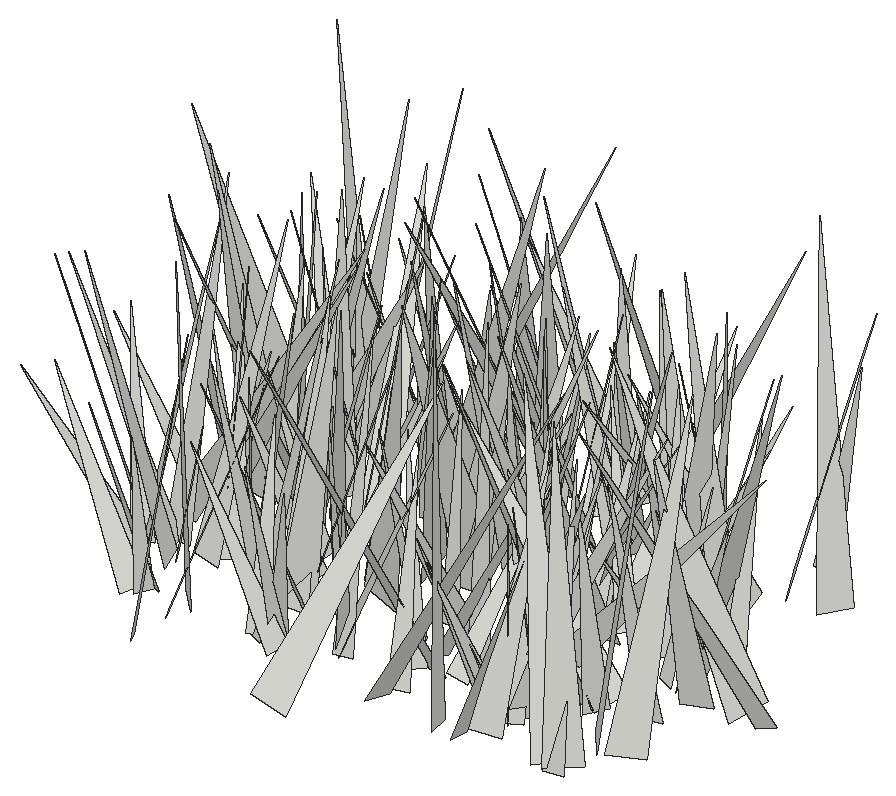
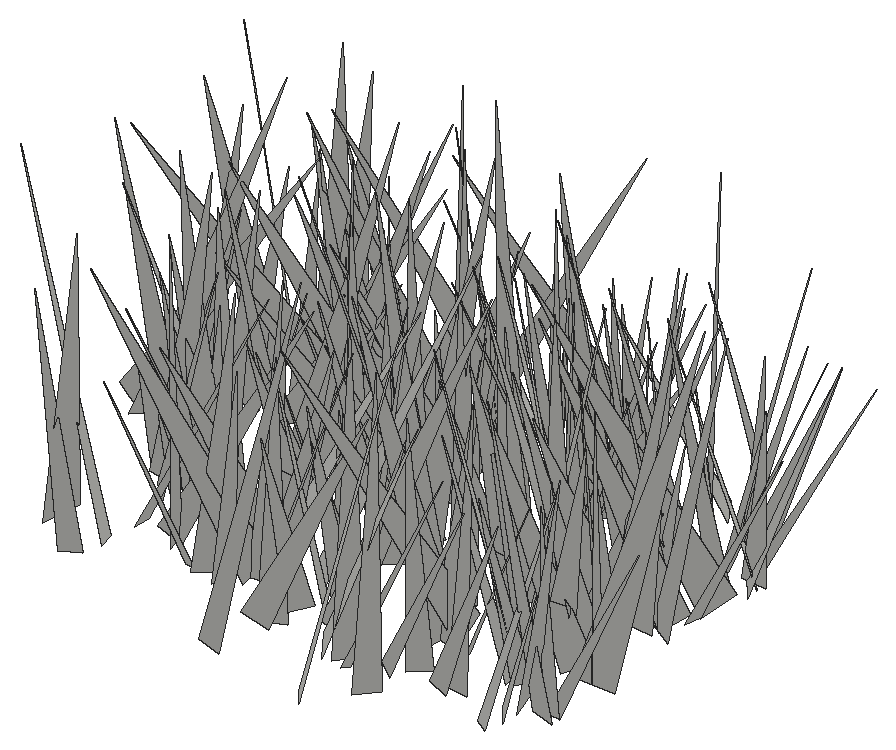
# SketchUp Ruby script. Lengths in inches.
U = 1.inch
M = Sketchup.active_model
def pt(a) = Geom::Point3d.new(a.map { |v| v * U })
def face(e, loops, mat)
  f = e.add_face(loops[0].map { |a| pt(a) })
  loops[1..].each { |l| e.add_face(l.map { |a| pt(a) }).erase! }
  f.material = f.back_material = mat if mat
  f
end
# faces: each face lists its corners as indices into pts; further lists are holes
def faces(e, pts, list, mat = nil) = list.each { |f| face(e, (f[0].is_a?(Array) ? f : [f]).map { |l| l.map { |i| pts[i] } }, mat) }
# xy, xz, yz: faces in a plane at the given z, y or x. An outline is a flat list of corners, or four numbers for a rectangle; further outlines are holes
def ring(l) = l.size == 4 ? [[l[0], l[1]], [l[2], l[1]], [l[2], l[3]], [l[0], l[3]]] : l.each_slice(2).to_a
def flat(e, list, mat, &to3) = list.each { |f| face(e, (f[0].is_a?(Array) ? f : [f]).map { |l| ring(l).map { |u, v| to3.(u, v) } }, mat) }
def xy(e, z, list, mat = nil) = flat(e, list, mat) { |x, y| [x, y, z] }
def xz(e, y, list, mat = nil) = flat(e, list, mat) { |x, z| [x, y, z] }
def yz(e, x, list, mat = nil) = flat(e, list, mat) { |y, z| [x, y, z] }
def lines(e, pts, list) = list.each { |a, b| e.add_line(pt(pts[a]), pt(pts[b])) }
# prism: a flat outline (further loops are holes) pulled along v
def prism(e, loops, v, mat = nil)
  f = face(e, loops, mat); d = Geom::Vector3d.new(v.map { |x| x * U })
  f.pushpull(f.normal.samedirection?(d) ? d.length : -d.length)
end
def box(e, o, s, mat = nil) = prism(e, [[o, [o[0] + s[0], o[1], o[2]], [o[0] + s[0], o[1] + s[1], o[2]], [o[0], o[1] + s[1], o[2]]]], [0, 0, s[2]], mat)
def at(x, y, z, deg = 0) = Geom::Transformation.translation(pt([x, y, z])) * Geom::Transformation.rotation(ORIGIN, Z_AXIS, deg.degrees)
def axes(o, x, y, z) = Geom::Transformation.new([*x, 0, *y, 0, *z, 0, *pt(o).to_a, 1])
def part(name) = M.definitions.add(name)
# library, detail: a bought-in or finely detailed component or shape, given as its bounding box
def library(name, o, s) = part(name).tap { |d| box(d.entities, o, s) }
def detail(e, o, s) = box(e.add_group.entities, o, s)
def put(e, d, t, mat = nil) = e.add_instance(d, t).tap { |i| i.material = mat if mat }
def group(e, t, mat = nil) = e.add_group.tap { |g| g.transformation = t; g.material = mat if mat }.entities
root = M.entities
c1 = part("fur_instance\#9")
p = [[0.8125,0,1.79],[0.67,-0.02,1.48],[0,-0.11,0],[0,0.11,0]]
faces(c1.entities,p,[[0,1,2,3]])
put(root,c1,axes([468.71,19.62,-21.86],[-0.73588,7.38124,0.25307],[6.98236,0.77818,-2.39362],[2.40696,-0.00075,7.02103]))
put(root,c1,axes([461.41,20.5,-21.86],[4.53649,3.63122,1.57008],[3.09166,-4.74451,2.04009],[-2.46831,0.73111,5.44092]))
put(root,c1,axes([466.3,23.18,-21.86],[-4.45422,0.97791,0.2811],[1.01486,4.3608,0.91044],[0.07343,-0.95002,4.4685]))
put(root,c1,axes([465.92,23.8125,-21.86],[-3.9744,-0.24759,1.6573],[0.13335,4.20562,0.94807],[1.67038,-0.92483,3.8676]))
put(root,c1,axes([459.53,23.55,-21.86],[2.92591,-1.89098,1.19539],[-1.88086,-3.14489,-0.37117],[-1.21125,0.31559,3.46396]))
put(root,c1,axes([465.51,24.1875,-21.86],[0.57309,-4.07864,0.58369],[-4.03575,-0.43699,0.90892],[0.82985,0.69149,4.01716]))
put(root,c1,axes([459.61,24.03,-21.86],[-2.05359,-3.75931,0.63579],[-3.81243,2.01617,-0.39286],[-0.04503,0.74602,4.26559]))
put(root,c1,axes([480.43,22.82,-21.86],[-4.52139,5.22079,2.42729],[5.56937,4.74843,0.161],[1.45961,-1.94607,6.90462]))
put(root,c1,axes([459.09,23.44,-21.86],[-3.88022,2.75048,0.41463],[2.75578,3.70465,1.21426],[-0.37781,-1.22622,4.59857]))
put(root,c1,axes([461.28,24.04,-21.86],[-4.9247,-5.05159,2.9073],[-5.39927,5.38751,0.21521],[2.19519,1.91829,7.05159]))
put(root,c1,axes([472.15,25.59,-21.86],[-3.80092,-6.72254,0.0507],[-6.48684,3.65215,-2.05545],[-1.76524,1.05421,7.4441]))
put(root,c1,axes([474.72,22.4,-21.86],[-7.45834,-2.27512,2.73301],[-2.96816,7.48025,-1.87304],[1.95846,2.67246,7.56933]))
put(root,c1,axes([476.37,24.59,-21.86],[-3.42009,-2.62307,1.97794],[-2.56254,3.91671,0.76324],[2.05575,0.51835,4.24205]))
put(root,c1,axes([479.86,22.92,-21.86],[-6.04844,4.67756,1.28768],[4.75602,6.12308,0.0974],[0.95811,-0.86582,7.6455]))
put(root,c1,axes([468,25.06,-21.86],[3.91592,-0.46866,0.80636],[-0.26131,-3.89224,-0.99321],[-0.89531,-0.91384,3.81675]))
put(root,c1,axes([476.48,23.02,-21.86],[-2.07384,5.25709,1.74566],[5.26815,2.4479,-1.11335],[1.712,-1.16445,5.54061]))
put(root,c1,axes([480.41,22.25,-21.86],[1.19098,5.93826,0.851],[5.76454,-1.37303,1.51343],[-1.66049,-0.50738,5.86438]))
put(root,c1,axes([474.43,25.75,-21.86],[-3.37943,-0.96857,0.84627],[-0.6019,3.29348,1.36586],[1.13667,-1.13567,3.23931]))
put(root,c1,axes([465.04,23.63,-21.86],[-1.62337,4.08317,1.17277],[4.21606,1.70273,-0.09236],[0.52201,-1.05424,4.39307]))
put(root,c1,axes([474.19,25.72,-21.86],[0.37183,-3.94608,0.38846],[-3.8933,-0.43727,-0.71534],[-0.75144,0.31297,3.89847]))
put(root,c1,axes([457.46,26.01,-21.86],[-4.70731,-0.314,0.0439],[-0.28456,4.4722,1.47573],[0.13983,-1.46975,4.48103]))
put(root,c1,axes([471.54,22.68,-21.86],[7.73901,0.54751,0.09462],[0.50511,-7.48314,1.98706],[-0.23147,1.9758,7.49957]))
put(root,c1,axes([475.8125,22.29,-21.86],[6.82922,2.21825,1.16198],[1.82522,-6.72015,2.10172],[-1.71447,1.68168,6.86597]))
put(root,c1,axes([471.79,23.63,-21.86],[-0.43977,4.5707,0.64422],[4.59918,0.3789,0.45132],[-0.39225,-0.6818,4.56957]))
put(root,c1,axes([461.29,22.77,-21.86],[4.51704,3.2359,0.24642],[3.07452,-4.40221,1.45028],[-1.0388,1.04161,5.3639]))
put(root,c1,axes([458.77,26.14,-21.86],[-6.28754,-2.52373,1.27093],[-2.51372,6.41179,0.29625],[1.29062,0.19325,6.76865]))
put(root,c1,axes([468,24.81,-21.86],[4.98455,3.49636,0.32674],[3.50629,-4.92427,-0.79656],[0.19289,-0.83908,6.03621]))
put(root,c1,axes([480.18,25.12,-21.86],[5.88152,4.86813,2.28116],[5.13014,-6.09312,-0.22398],[-1.60749,-1.63397,7.63157]))
put(root,c1,axes([463.08,26.35,-21.86],[-4.89796,-0.50596,1.28828],[-0.38248,5.0478,0.52832],[1.33018,-0.4116,4.8956]))
put(root,c1,axes([458.69,26.64,-21.86],[3.46775,1.51161,0.84573],[1.722,-3.21287,-1.3182],[-0.18693,-1.55498,3.54578]))
put(root,c1,axes([464.76,26.21,-21.86],[2.84119,-6.18581,2.36185],[-6.62137,-2.65127,1.02137],[0.00779,2.57322,6.73004]))
put(root,c1,axes([467.27,25.84,-21.86],[1.82668,3.73793,1.95155],[3.99067,-2.21946,0.51574],[-1.36206,-1.48974,4.1283]))
put(root,c1,axes([476.17,26.43,-21.86],[-3.08736,-2.6391,1.38175],[-2.74426,3.29386,0.15946],[1.15895,0.7691,4.05847]))
put(root,c1,axes([464.96,23.41,-21.86],[4.10406,6.33899,0.98584],[6.11766,-4.2195,1.66374],[-1.93105,0.10466,7.36601]))
put(root,c1,axes([465.36,26.02,-21.86],[-3.16767,-3.69393,0.44061],[-3.42422,2.66901,-2.24153],[-1.45395,1.76199,4.31912]))
put(root,c1,axes([478.11,27.0625,-21.86],[-4.08084,-6.31933,0.93728],[-6.28934,3.77891,-1.90517],[-1.12095,1.80323,7.27719]))
put(root,c1,axes([470.4,26.77,-21.86],[-4.55771,-1.35516,1.4154],[-1.26006,4.77117,0.51063],[1.50069,-0.10962,4.72742]))
put(root,c1,axes([471.85,28.2,-21.86],[1.26749,-5.25605,0.55346],[-5.00773,-1.37633,-1.60227],[-1.68968,0.13629,5.16385]))
put(root,c1,axes([476.68,24.78,-21.86],[4.97283,-0.90694,1.68915],[-1.45035,-4.85051,1.66547],[-1.25389,2.01364,4.77261]))
put(root,c1,axes([478.7,26.98,-21.86],[3.6689,-2.8215,1.45683],[-2.81207,-3.92099,-0.512],[-1.47496,0.45716,4.59995]))
put(root,c1,axes([470.6875,24.8125,-21.86],[5.2038,5.70361,2.35891],[5.67233,-5.63566,1.11317],[-2.43315,-0.93989,7.64013]))
put(root,c1,axes([474.21,28.54,-21.86],[1.01842,-6.5564,0.3467],[-5.92672,-0.76709,2.90332],[2.82498,0.75429,5.9661]))
put(root,c1,axes([466.95,28.66,-21.86],[-0.13317,-8.12567,1.45261],[-7.87911,0.55826,2.40046],[2.46092,1.34765,7.76415]))
put(root,c1,axes([468.55,24.32,-21.86],[1.43264,6.02249,0.66756],[5.77311,-1.565,1.72927],[-1.84042,-0.22107,5.94411]))
put(root,c1,axes([471.28,25.3125,-21.86],[-4.35702,1.54483,0.37411],[1.45493,4.3157,-0.87633],[0.64002,0.7059,4.53896]))
put(root,c1,axes([476.74,24.23,-21.86],[-5.37291,2.30629,0.61766],[1.96946,5.14098,-2.06404],[1.34972,1.6793,5.47055]))
put(root,c1,axes([457.12,26.87,-21.86],[-4.61833,-3.74237,0.73758],[-3.79853,4.40694,-1.4242],[-0.34716,1.56584,5.77113]))
put(root,c1,axes([476.65,26.6875,-21.86],[2.40837,2.51325,1.53163],[2.71206,-2.66382,0.10655],[-1.14326,-1.0248,3.47927]))
put(root,c1,axes([481.76,24.96,-21.86],[-4.86903,5.31705,1.90275],[5.12727,5.21523,-1.45307],[2.36698,-0.35954,7.06166]))
put(root,c1,axes([464.75,25.98,-21.86],[-0.45657,6.34549,1.8425],[6.59681,0.54314,-0.23589],[0.37708,-1.81886,6.35752]))
put(root,c1,axes([458.1875,27.12,-21.86],[-6.00367,-1.40851,0.07652],[-1.40991,5.98159,-0.51624],[-0.04369,0.52005,6.14503]))
put(root,c1,axes([464.02,28.47,-21.86],[-4.35378,0.44066,1.23045],[0.84047,4.2213,1.46212],[1.0009,-1.62788,4.12453]))
put(root,c1,axes([461.8,27.29,-21.86],[3.22406,2.21993,1.84513],[2.48282,-3.54361,-0.0749],[-1.47248,-1.11442,3.91371]))
put(root,c1,axes([480.71,27.74,-21.86],[-0.10037,-5.00985,1.67679],[-5.24561,-0.10471,-0.62683],[-0.62754,1.67652,4.9715]))
put(root,c1,axes([478.71,27.92,-21.86],[-6.39943,2.86094,0.01202],[2.71801,6.07041,2.2137],[-0.89308,-2.0256,6.65111]))
put(root,c1,axes([475.84,25.44,-21.86],[5.89458,-2.32049,1.52507],[-2.76984,-5.16651,2.8446],[-0.1962,3.22166,5.6603]))
put(root,c1,axes([457.125,26.49,-21.86],[-0.91318,4.58049,0.90258],[4.61205,0.74242,0.89849],[-0.72428,-1.04754,4.5834]))
put(root,c1,axes([472.99,25.71,-21.86],[-0.63847,4.33122,0.11328],[4.14955,0.64421,-1.24344],[1.2464,0.07394,4.19773]))
put(root,c1,axes([475.76,26.43,-21.86],[6.0984,-4.54505,0.22334],[-3.82324,-4.91501,4.37303],[2.46783,3.61705,6.22291]))
put(root,c1,axes([474.74,28.15,-21.86],[-2.40754,3.72637,1.88833],[4.14407,2.40561,0.53634],[0.52762,-1.89079,4.40391]))
put(root,c1,axes([471.41,26.62,-21.86],[5.44463,0.12063,0.24069],[0.04962,-5.23956,1.50366],[-0.26462,1.49964,5.23426]))
put(root,c1,axes([481.4,29.7,-21.86],[1.80262,-6.00522,1.15434],[-6.08405,-1.88243,-0.2921],[-0.61598,1.01901,6.26312]))
put(root,c1,axes([461.55,27.88,-21.86],[5.12051,1.66894,1.66295],[1.70709,-5.37015,0.13306],[-1.62376,-0.38277,5.38398]))
put(root,c1,axes([475.67,29.83,-21.86],[-0.04463,-6.97717,1.39975],[-6.92736,-0.27772,-1.60522],[-1.62845,1.37265,6.79015]))
put(root,c1,axes([472.74,27.31,-21.86],[1.55743,6.34801,1.89562],[6.44853,-1.89902,1.06134],[-1.51893,-1.55328,6.44953]))
put(root,c1,axes([461.53,28.84,-21.86],[3.75751,0.05108,0.3502],[0.07903,-3.76142,-0.29936],[-0.34497,-0.30538,3.74592]))
put(root,c1,axes([457.42,26.09,-21.86],[4.3588,4.87451,1.02077],[4.50794,-4.43827,1.9448],[-2.11691,0.58556,6.24322]))
put(root,c1,axes([484.52,30.01,-21.86],[-2.35699,-6.63901,0.53799],[-6.01099,1.87426,-3.2057],[-2.86948,1.52709,6.27339]))
put(root,c1,axes([459.84,26.93,-21.86],[1.8777,6.7714,0.98346],[6.8334,-1.90815,0.09124],[-0.35155,-0.923,7.02632]))
put(root,c1,axes([476.92,29.68,-21.86],[-2.69174,-3.80387,0.07847],[-3.66679,2.56798,-1.29661],[-1.01502,0.8106,4.47591]))
put(root,c1,axes([465.24,27.73,-21.86],[3.15484,4.86518,0.39731],[4.85003,-3.07066,-0.91053],[0.55227,-0.82578,5.72659]))
put(root,c1,axes([463.25,29.71,-21.86],[5.75664,2.23558,0.62086],[2.31995,-5.52205,-1.62697],[0.03364,-1.74108,5.95732]))
put(root,c1,axes([459.24,28.82,-21.86],[-4.37143,-2.8181,2.86453],[-3.24687,4.97094,-0.06453],[2.3675,1.61389,5.20067]))
put(root,c1,axes([475.4375,27.93,-21.86],[1.4103,3.34023,0.25009],[3.32818,-1.428,0.30438],[-0.37801,-0.11091,3.61295]))
put(root,c1,axes([462.52,31.6,-21.86],[-2.5118,-6.70095,1.69222],[-6.07027,2.9998,2.86854],[3.30427,0.41708,6.55616]))
put(root,c1,axes([461.86,30.82,-21.86],[0.42063,-4.67833,0.35233],[-4.37367,-0.26302,1.72907],[1.69763,0.48155,4.36738]))
put(root,c1,axes([483.22,30.54,-21.86],[-7.69272,2.37823,1.5322],[2.71051,7.46743,2.01798],[0.8104,-2.40066,7.79498]))
put(root,c1,axes([475.38,31.59,-21.86],[-0.92127,-7.60318,0.93237],[-7.64439,0.85236,-0.60268],[-0.49091,0.99576,7.63504]))
put(root,c1,axes([463.26,29.9,-21.86],[-4.01235,0.08097,0.58825],[0.14386,4.03101,0.42638],[0.5761,-0.44265,3.99045]))
put(root,c1,axes([458.06,27.42,-21.86],[1.84085,7.01016,1.12106],[6.97031,-2.00445,1.08846],[-1.34679,-0.79226,7.16563]))
put(root,c1,axes([470.19,28.74,-21.86],[0.81104,4.54834,1.26147],[4.65262,-0.98593,0.56355],[-0.7949,-1.13006,4.58559]))
put(root,c1,axes([474.23,29.82,-21.86],[3.78368,4.97369,3.03573],[5.56614,-4.15585,-0.12867],[-1.72376,-2.50217,6.24798]))
put(root,c1,axes([460.62,27.62,-21.86],[-4.8792,2.06982,0.10093],[1.96371,4.70056,-1.46614],[0.66196,1.31208,5.09325]))
put(root,c1,axes([465.62,29.98,-21.86],[4.19942,-1.36084,1.21546],[-1.38514,-4.36301,-0.09922],[-1.1877,0.2767,4.41329]))
put(root,c1,axes([457.09,30.25,-21.86],[-4.32306,0.06447,0.02072],[0.06687,4.27292,0.65655],[0.01068,-0.65679,4.2734]))
put(root,c1,axes([466.99,31.83,-21.86],[7.73874,0.04549,1.82687],[0.5794,-7.60007,-2.26513],[-1.73315,-2.33761,7.39995]))
put(root,c1,axes([474.72,27.8125,-21.86],[5.53562,0.75174,0.06867],[0.66774,-5.11345,2.14935],[-0.35205,2.12143,5.1564]))
put(root,c1,axes([468.03,33.12,-21.86],[6.63906,-4.24471,1.17982],[-3.75911,-6.57064,-2.48644],[-2.29753,-1.51516,7.47745]))
put(root,c1,axes([458.01,30.49,-21.86],[1.53162,3.70831,1.75315],[4.01532,-0.97314,-1.44953],[0.83802,-2.1148,3.74116]))
put(root,c1,axes([459.33,29.61,-21.86],[0.68239,3.8164,1.4602],[3.78451,-1.14857,1.23331],[-1.54098,-1.13076,3.67553]))
put(root,c1,axes([457.02,28.76,-21.86],[6.90826,-2.9112,0.5406],[-2.88435,-6.30625,2.89882],[0.66922,2.87186,6.91346]))
put(root,c1,axes([474.66,28.65,-21.86],[-6.55431,0.09701,1.7896],[-0.34688,6.588,-1.62754],[1.75834,1.66126,6.34976]))
put(root,c1,axes([480.05,32.08,-21.86],[-4.12038,-2.11418,1.50488],[-1.47976,4.23386,1.89649],[2.13184,-1.14743,4.225]))
put(root,c1,axes([464.02,29.4375,-21.86],[3.98122,4.30027,2.75674],[4.211,-4.74141,1.31475],[-2.89126,-0.98426,5.71085]))
put(root,c1,axes([469.1875,31.34,-21.86],[2.1882,-4.93746,0.79161],[-4.93819,-1.99768,1.19031],[0.78701,1.19336,5.26781]))
put(root,c1,axes([472.71,29.99,-21.86],[-3.32037,-5.8988,2.51801],[-6.36421,2.67847,-2.11746],[-0.7956,3.19234,6.42939]))
put(root,c1,axes([458.375,32,-21.86],[-0.95753,-7.17721,1.84222],[-7.39469,1.0444,0.22542],[0.47406,1.79439,7.23729]))
put(root,c1,axes([476.42,33.21,-21.86],[-2.58943,-3.13022,0.07236],[-2.65217,2.2427,2.10831],[1.66419,-1.2964,3.47253]))
put(root,c1,axes([465.69,28.2,-21.86],[5.66789,4.81372,1.80284],[4.22946,-5.89252,2.43659],[-2.92126,0.80836,7.02566]))
put(root,c1,axes([460.14,32.66,-21.86],[-3.16334,-6.14078,0.476],[-6.132,3.08971,-0.89149],[-0.57823,0.82883,6.8499]))
put(root,c1,axes([479.23,31.74,-21.86],[2.31724,-3.70248,0.25487],[-3.62607,-2.19471,1.08527],[0.79054,0.78602,4.23086]))
put(root,c1,axes([457.45,31.75,-21.86],[-3.32824,-5.52708,1.61735],[-5.74671,3.30884,-0.51825],[0.37393,1.65668,6.43096]))
put(root,c1,axes([479.375,30.31,-21.86],[1.79566,3.71313,0.76849],[3.77743,-1.82574,-0.00496],[-0.33004,-0.69403,4.12452]))
put(root,c1,axes([469.39,31.23,-21.86],[5.13352,5.29295,1.04527],[5.31008,-4.70157,-2.27141],[0.95446,-2.31104,7.01492]))
put(root,c1,axes([460.97,32.6,-21.86],[5.69332,3.04756,1.30745],[3.31373,-5.12843,-2.47574],[0.12746,-2.79687,5.96424]))
put(root,c1,axes([457.47,30.84,-21.86],[6.30652,-2.10429,0.15189],[-2.07978,-6.12031,1.56194],[0.35446,1.52876,6.46224]))
put(root,c1,axes([468.78,32.21,-21.86],[1.64053,-3.56149,0.70323],[-3.59089,-1.47867,0.88831],[0.53314,0.99969,3.81922]))
put(root,c1,axes([458.93,32.69,-21.86],[6.73753,-0.02978,4.19134],[0.53715,-7.86314,-0.91932],[-4.15689,-1.06433,6.67458]))
put(root,c1,axes([470.29,32.58,-21.86],[4.81176,-1.3762,1.70282],[-1.26945,-5.10354,-0.53746],[-1.78382,-0.0803,4.97575]))
put(root,c1,axes([478.27,31.95,-21.86],[-2.39493,4.93051,2.15105],[5.27679,2.61079,-0.10925],[1.04521,-1.88321,5.4803]))
put(root,c1,axes([479.87,30.4,-21.86],[5.27233,3.79468,0.9806],[3.62511,-5.34626,1.19781],[-1.48988,0.42019,6.38454]))
put(root,c1,axes([467.375,33.375,-21.86],[0.9927,-7.18833,2.00129],[-7.23058,-0.4281,2.04891],[1.84279,2.19257,6.96128]))
put(root,c1,axes([468.27,31.86,-21.86],[4.34648,-1.55951,0.20323],[-1.53377,-4.07129,1.56122],[0.34774,1.53551,4.34586]))
put(root,c1,axes([476.65,34.55,-21.86],[0.33482,-6.22736,0.74708],[-6.26175,-0.28913,0.39628],[0.3585,0.76592,6.22375]))
put(root,c1,axes([473.92,33.28,-21.86],[6.64605,0.23955,0.93352],[0.28653,-6.70181,-0.32012],[-0.92019,-0.35664,6.64266]))
put(root,c1,axes([464.67,34.58,-21.86],[0.91835,-4.65892,0.5996],[-4.68613,-0.86646,0.44487],[0.32448,0.67241,4.72768]))
put(root,c1,axes([461.3,34.88,-21.86],[-4.71687,-4.84842,1.35584],[-4.8132,4.8877,0.73342],[1.47602,0.44449,6.72444]))
put(root,c1,axes([478.5625,34.09,-21.86],[7.28234,-1.08518,0.65082],[-1.04869,-7.30325,-0.44316],[-0.70811,-0.34428,7.3494]))
put(root,c1,axes([474.49,31.81,-21.86],[-3.28423,2.60896,0.74342],[2.31234,3.30268,-1.37511],[1.4186,0.65664,3.96257]))
put(root,c1,axes([475.73,32.51,-21.86],[-4.1604,2.35856,0.20079],[2.33408,4.15517,-0.44576],[0.39395,0.28953,4.76162]))
put(root,c1,axes([477.88,33.38,-21.86],[-2.17723,3.86998,1.04919],[4.00343,2.16477,0.32287],[0.22393,-1.07466,4.42864]))
put(root,c1,axes([460.27,34.4,-21.86],[-4.38219,4.14776,3.28171],[4.71988,4.98997,-0.0042],[2.38668,-2.25242,6.03386]))
put(root,c1,axes([474.41,32.31,-21.86],[-4.0426,1.99311,1.15136],[1.52694,4.06338,-1.67276],[1.72237,1.07573,4.18533]))
put(root,c1,axes([473.24,32.25,-21.86],[1.74005,3.73475,0.21366],[3.48509,-1.70407,1.40429],[-1.35946,0.41179,3.87351]))
put(root,c1,axes([460.89,30.79,-21.86],[-5.84983,3.65343,0.11485],[3.32744,5.4123,-2.68634],[1.51292,2.22277,6.35229]))
put(root,c1,axes([476.29,35.34,-21.86],[4.71855,-5.46855,1.25045],[-5.59838,-4.69426,0.59612],[-0.35606,1.33873,7.19821]))
put(root,c1,axes([462.04,34.47,-21.86],[4.56637,-2.19972,0.30987],[-2.21681,-4.46657,0.96025],[0.14341,0.99877,4.97679]))
put(root,c1,axes([457.99,33.93,-21.86],[0.08928,4.21713,1.27448],[4.4055,-0.088,-0.01741],[-0.00879,-1.27457,4.21804]))
put(root,c1,axes([468.73,33.9,-21.86],[-0.20342,5.45726,1.92359],[5.57072,0.70526,-1.41173],[1.56492,-1.80117,5.27542]))
put(root,c1,axes([479.375,34.17,-21.86],[-0.80473,7.1427,2.6366],[7.51279,0.31449,1.44102],[-1.23607,-2.73867,7.04196]))
put(root,c1,axes([458.24,34.42,-21.86],[3.99026,4.07334,2.14881],[4.32029,-4.29562,0.12027],[-1.59518,-1.44473,5.70086]))
put(root,c1,axes([456.92,36.42,-21.86],[1.74253,-7.39949,2.19817],[-7.33714,-2.28781,-1.88496],[-2.39807,1.62304,7.36449]))
put(root,c1,axes([471.21,33.73,-21.86],[-0.87591,3.86506,0.33078],[3.84564,0.82067,0.59405],[-0.50909,-0.4507,3.91829]))
put(root,c1,axes([460.95,34.05,-21.86],[-3.88558,0.60859,0.85055],[0.43871,3.91906,-0.80001],[0.9494,0.67978,3.85072]))
put(root,c1,axes([470.14,36.57,-21.86],[-5.60021,-5.8066,0.30959],[-5.79691,5.54128,-0.92996],[-0.45638,0.8674,8.01337]))
put(root,c1,axes([478.99,35.14,-21.86],[-4.01127,-3.66818,1.32519],[-3.89401,3.87381,-1.06408],[0.2199,1.68524,5.33044]))
put(root,c1,axes([473.25,34.55,-21.86],[-6.43148,-3.95381,0.27263],[-3.76371,5.93049,-2.78112],[-1.24153,2.50351,7.01869]))
put(root,c1,axes([476.67,37.41,-21.86],[0.43766,-5.35462,0.13989],[-4.92597,-0.45748,-2.09965],[-2.10387,-0.04276,4.94519]))
put(root,c1,axes([480.51,33.07,-21.86],[-4.48023,1.71415,0.10108],[1.53614,4.12726,-1.90446],[0.76734,1.74596,4.4027]))
put(root,c1,axes([475.76,34.84,-21.86],[2.80072,3.68056,0.20092],[3.50306,-2.57922,-1.58339],[1.14693,-1.10998,4.34551]))
put(root,c1,axes([458.45,34.61,-21.86],[6.19902,-0.22924,1.58295],[-0.50577,-6.29178,1.06951],[-1.51739,1.16065,6.11037]))
put(root,c1,axes([458.21,35.79,-21.86],[4.35594,-4.3452,0.48537],[-4.22774,-4.01128,2.03138],[1.11472,1.7662,5.80763]))
put(root,c1,axes([463.12,33.17,-21.86],[-3.48559,6.14429,0.41822],[6.11379,3.5101,-0.61419],[0.74073,-0.05879,7.03735]))
put(root,c1,axes([463.61,37.34,-21.86],[-1.87294,-5.65903,1.00828],[-5.62978,2.02003,0.87988],[1.16052,0.66634,5.89562]))
put(root,c1,axes([457.27,35.8,-21.86],[-4.85936,-1.80324,2.4582],[-1.94231,5.39639,0.11902],[2.34986,0.73149,5.18178]))
put(root,c1,axes([468.29,36.04,-21.86],[-3.7574,-4.18768,1.74578],[-4.4509,3.84178,-0.36412],[0.87968,1.55129,5.61445]))
put(root,c1,axes([478.11,37.3125,-21.86],[-5.4104,-1.19331,0.05848],[-1.15989,5.3113,1.06983],[0.28647,-1.03242,5.43616]))
put(root,c1,axes([477.49,34.84,-21.86],[5.18015,0.30458,2.40247],[-0.20645,-5.59667,1.15468],[-2.41288,1.13276,5.059]))
put(root,c1,axes([459.87,34.95,-21.86],[-2.82943,5.24506,0.49337],[5.22615,2.72388,1.01368],[-0.66438,-0.91081,5.87271]))
put(root,c1,axes([471.94,38.03,-21.86],[-1.23587,-5.65616,0.92472],[-5.5483,1.41785,1.25724],[1.43652,0.61007,5.65145]))
put(root,c1,axes([467.24,39.26,-21.86],[-0.88458,-7.33954,0.10795],[-7.20369,0.84713,-1.43254],[-1.40973,0.27658,7.25253]))
put(root,c1,axes([459.22,37.26,-21.86],[1.41484,-4.55258,1.06253],[-4.54528,-1.07998,1.42506],[1.09333,1.40157,4.54939]))
put(root,c1,axes([469.53,35.33,-21.86],[3.33394,1.47543,1.26624],[0.9738,-3.44268,1.44745],[-1.68284,0.93087,3.34618]))
put(root,c1,axes([471.8,37.05,-21.86],[0.51311,-4.91857,2.52241],[-5.22585,-1.25725,-1.38854],[-1.80151,2.24614,4.74633]))
put(root,c1,axes([474.5,34.56,-21.86],[-2.9389,4.8588,0.20427],[4.55933,2.83593,-1.85926],[1.6918,0.79774,5.36547]))
put(root,c1,axes([476.21,37.63,-21.86],[5.47086,1.91538,2.35531],[2.21322,-5.83902,-0.39241],[-2.07794,-1.17628,5.78316]))
put(root,c1,axes([461.99,37.83,-21.86],[-3.92921,-1.09616,0.24918],[-1.11465,3.91653,-0.34741],[0.14562,0.40197,4.06442]))
put(root,c1,axes([468.09,37.52,-21.86],[2.99214,-2.75371,1.44433],[-3.06357,-2.95389,0.71483],[-0.53251,1.52102,4.0031]))
put(root,c1,axes([463.61,37.01,-21.86],[7.18053,-1.42617,1.70446],[-1.71997,-7.21687,1.20732],[-1.40743,1.54336,7.22055]))
put(root,c1,axes([469.01,37.62,-21.86],[4.26525,2.34746,1.0733],[2.44325,-4.34035,-0.2164],[-0.83252,-0.71113,4.86375]))
put(root,c1,axes([459.65,38.01,-21.86],[4.85217,1.44436,0.49792],[1.4914,-4.83766,-0.50049],[-0.33141,-0.62336,5.03778]))
put(root,c1,axes([473.77,38.76,-21.86],[3.82096,-4.05561,2.24215],[-4.19487,-4.26194,-0.56033],[-1.96935,1.20949,5.5438]))
put(root,c1,axes([472.15,37.02,-21.86],[-6.83624,-2.0461,0.45627],[-2.08301,6.45462,-2.26447],[-0.23611,2.29788,6.76704]))
put(root,c1,axes([459.06,38.05,-21.86],[2.18192,-3.03993,1.35648],[-3.32882,-1.9865,0.90262],[0.01238,1.6293,3.63142]))
put(root,c1,axes([478.28,39.25,-21.86],[7.20484,3.15988,1.15153],[3.35999,-6.88107,-2.14053],[-0.14588,-2.42624,7.57051]))
put(root,c1,axes([462.74,39.6875,-21.86],[2.83156,-3.99697,0.33188],[-4.00855,-2.80696,0.39506],[0.13188,0.49882,4.88236]))
put(root,c1,axes([456.8,38.87,-21.86],[-2.53868,-3.44184,0.53172],[-3.38696,2.28677,-1.36858],[-0.81085,1.22404,4.05193]))
put(root,c1,axes([460.01,37.11,-21.86],[5.71474,5.0925,1.62445],[5.00095,-5.93344,1.00766],[-1.88756,-0.30227,7.58791]))
put(root,c1,axes([466.49,39.82,-21.86],[-1.9055,-4.08481,0.78377],[-4.15591,1.83492,-0.5407],[-0.16841,0.93717,4.47485]))
put(root,c1,axes([460.66,40.06,-21.86],[-1.39495,-5.41554,1.57218],[-5.52882,1.63221,0.71678],[1.10996,1.3242,5.54619]))
put(root,c1,axes([456.75,39.25,-21.86],[-0.60793,-4.00143,1.69165],[-4.28266,0.83877,0.44495],[0.72934,1.58988,4.02282]))
put(root,c1,axes([465.43,40.64,-21.86],[5.78336,-2.78291,1.02515],[-2.6557,-5.85961,-0.92463],[-1.32013,-0.40388,6.35113]))
put(root,c1,axes([474.6,38.79,-21.86],[2.24479,3.42751,0.35228],[3.3467,-2.06895,-1.19586],[0.81948,-0.93948,3.91878]))
put(root,c1,axes([472.98,38.75,-21.86],[-4.87312,1.26006,1.29377],[1.19613,5.04128,-0.40455],[1.35309,0.08157,5.01711]))
put(root,c1,axes([463.23,36.12,-21.86],[7.74445,1.42991,0.81828],[1.0012,-7.20795,3.11989],[-1.30836,2.94814,7.231]))
put(root,c1,axes([465.12,41.19,-21.86],[-3.99864,-1.03805,0.42764],[-0.78188,3.71014,1.695],[0.80565,-1.55139,3.76744]))
put(root,c1,axes([472.35,37.58,-21.86],[7.35163,-0.33714,0.71191],[-0.54127,-7.01692,2.26646],[-0.57229,2.30568,7.00167]))
put(root,c1,axes([458.28,41.53,-21.86],[-3.01664,-4.03882,0.35129],[-3.9528,3.02747,0.86334],[0.90049,-0.2406,4.96657]))
put(root,c1,axes([469.4375,40.25,-21.86],[1.77747,-4.94769,1.74658],[-5.22789,-1.82695,0.145],[-0.44649,1.69476,5.25529]))
put(root,c1,axes([463.79,40.43,-21.86],[-2.18116,-3.44946,0.52539],[-3.41914,1.9894,-1.13316],[-0.6959,1.0372,3.92074]))
put(root,c1,axes([456.88,39.61,-21.86],[2.76981,6.05425,2.08045],[6.39697,-2.70498,-0.64491],[-0.24704,-2.16406,6.62646]))
put(root,c1,axes([461.4,40.3,-21.86],[-0.15517,3.72025,1.9318],[3.94772,-0.52047,1.31942],[-1.40985,-1.86683,3.48188]))
put(root,c1,axes([470.05,40.56,-21.86],[-2.55985,4.83206,1.74885],[4.89019,1.69025,2.4878],[-1.579,-2.59892,4.86955]))
put(root,c1,axes([480.9,38.71,-21.86],[-7.32985,2.37013,1.25415],[2.21242,7.40801,-1.06942],[1.51512,0.64882,7.62892]))
put(root,c1,axes([478.81,40.76,-21.86],[0.64184,-5.02818,1.67754],[-5.1921,-0.25617,1.21871],[1.0672,1.77778,4.9203]))
put(root,c1,axes([463.23,42.28,-21.86],[5.82388,-2.11588,0.96568],[-1.89422,-5.82584,-1.34106],[-1.34958,-0.95373,6.04946]))
put(root,c1,axes([469.28,38.78,-21.86],[-3.56448,3.67904,0.44666],[3.56023,3.5714,-1.00507],[1.02934,0.38746,5.02301]))
put(root,c1,axes([466.8125,40.48,-21.86],[-5.23852,-3.39609,0.6769],[-3.443,4.97658,-1.67721],[-0.37061,1.77027,6.01352]))
put(root,c1,axes([470.18,43.18,-21.86],[-2.86218,-6.85746,0.77217],[-6.83354,2.93291,0.71683],[0.96112,0.43167,7.39614]))
put(root,c1,axes([458.15,40.41,-21.86],[-3.1769,-1.92196,0.83625],[-2.09296,2.82701,-1.45378],[-0.11299,1.67333,3.4166]))
put(root,c1,axes([458.21,38.77,-21.86],[-7.80069,-0.47128,0.71432],[-0.70737,7.23754,-2.94972],[0.48165,2.99651,7.23686]))
put(root,c1,axes([465.05,44.13,-21.86],[-6.10663,-5.12788,1.30944],[-4.81653,6.21333,1.86984],[2.19336,-0.63253,7.75176]))
